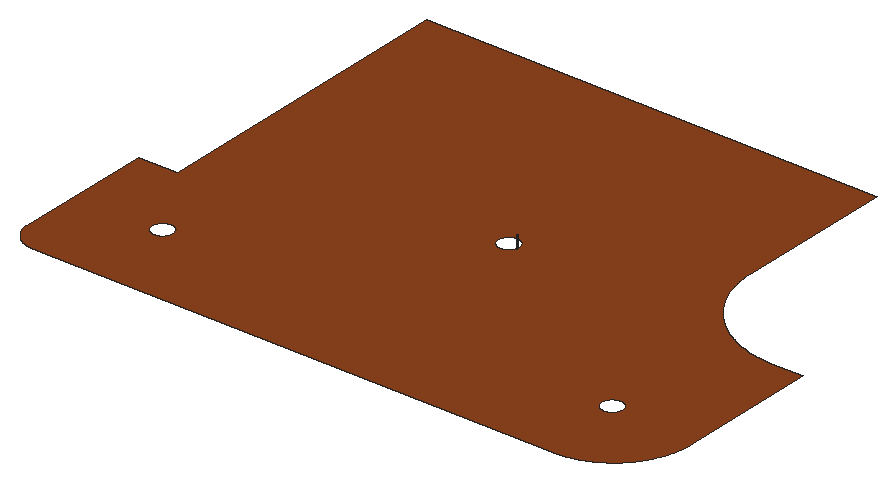
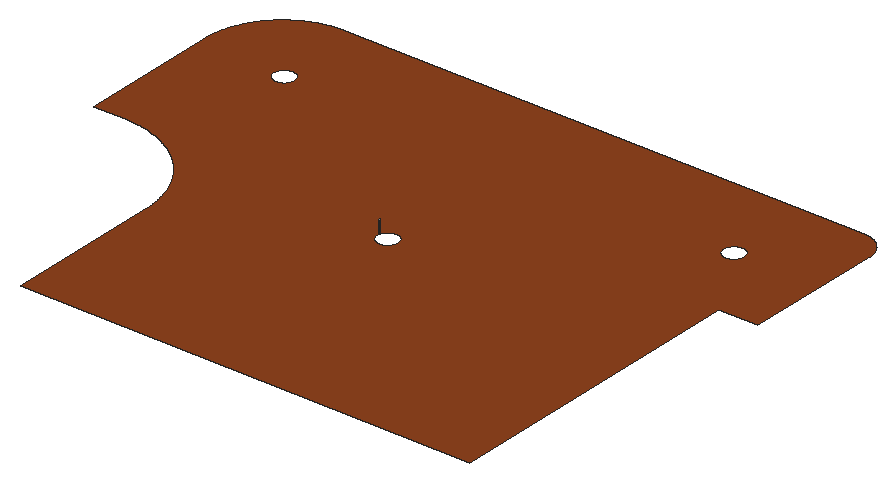
# SketchUp Ruby script. Lengths in inches.
U = 1.inch
M = Sketchup.active_model
def pt(a) = Geom::Point3d.new(a.map { |v| v * U })
def face(e, loops, mat)
  f = e.add_face(loops[0].map { |a| pt(a) })
  loops[1..].each { |l| e.add_face(l.map { |a| pt(a) }).erase! }
  f.material = f.back_material = mat if mat
  f
end
# faces: each face lists its corners as indices into pts; further lists are holes
def faces(e, pts, list, mat = nil) = list.each { |f| face(e, (f[0].is_a?(Array) ? f : [f]).map { |l| l.map { |i| pts[i] } }, mat) }
# xy, xz, yz: faces in a plane at the given z, y or x. An outline is a flat list of corners, or four numbers for a rectangle; further outlines are holes
def ring(l) = l.size == 4 ? [[l[0], l[1]], [l[2], l[1]], [l[2], l[3]], [l[0], l[3]]] : l.each_slice(2).to_a
def flat(e, list, mat, &to3) = list.each { |f| face(e, (f[0].is_a?(Array) ? f : [f]).map { |l| ring(l).map { |u, v| to3.(u, v) } }, mat) }
def xy(e, z, list, mat = nil) = flat(e, list, mat) { |x, y| [x, y, z] }
def xz(e, y, list, mat = nil) = flat(e, list, mat) { |x, z| [x, y, z] }
def yz(e, x, list, mat = nil) = flat(e, list, mat) { |y, z| [x, y, z] }
def lines(e, pts, list) = list.each { |a, b| e.add_line(pt(pts[a]), pt(pts[b])) }
# prism: a flat outline (further loops are holes) pulled along v
def prism(e, loops, v, mat = nil)
  f = face(e, loops, mat); d = Geom::Vector3d.new(v.map { |x| x * U })
  f.pushpull(f.normal.samedirection?(d) ? d.length : -d.length)
end
def box(e, o, s, mat = nil) = prism(e, [[o, [o[0] + s[0], o[1], o[2]], [o[0] + s[0], o[1] + s[1], o[2]], [o[0], o[1] + s[1], o[2]]]], [0, 0, s[2]], mat)
def at(x, y, z, deg = 0) = Geom::Transformation.translation(pt([x, y, z])) * Geom::Transformation.rotation(ORIGIN, Z_AXIS, deg.degrees)
def axes(o, x, y, z) = Geom::Transformation.new([*x, 0, *y, 0, *z, 0, *pt(o).to_a, 1])
def part(name) = M.definitions.add(name)
# library, detail: a bought-in or finely detailed component or shape, given as its bounding box
def library(name, o, s) = part(name).tap { |d| box(d.entities, o, s) }
def detail(e, o, s) = box(e.add_group.entities, o, s)
def put(e, d, t, mat = nil) = e.add_instance(d, t).tap { |i| i.material = mat if mat }
def group(e, t, mat = nil) = e.add_group.tap { |g| g.transformation = t; g.material = mat if mat }.entities
root = M.entities
M.materials.add("[Wood Fence]").color = [142, 67, 30]
xy(root,242,[[[21.02,135.92,20.92,135.93,20.6875,135.93,20.61,135.9375,20.53,135.94,20.29,135.97,20.22,135.98,20.14,135.99,20.0625,136,19.98,136.01,19.91,136.02,19.75,136.06,19.68,136.07,19.52,136.11,19.45,136.13,19.37,136.15,19.3,136.17,19.22,136.19,19.15,136.22,19.07,136.24,19,136.27,18.92,136.3,18.85,136.32,18.78,136.35,18.7,136.38,18.56,136.44,18.49,136.48,18.35,136.54,18.28,136.58,18.21,136.61,17.93,136.77,17.87,136.81,17.73,136.89,17.67,136.9375,17.6,136.98,17.54,137.02,17.47,137.07,17.41,137.12,17.35,137.16,17.29,137.21,17.22,137.26,17.16,137.3125,17.1,137.36,17.04,137.41,16.99,137.47,16.87,137.57,16.8125,137.625,16.76,137.68,16.59,137.85,16.49,137.97,16.4375,138.03,16.39,138.09,16.19,138.33,16.15,138.4,16.1,138.46,16.06,138.53,16.01,138.59,15.97,138.66,15.93,138.72,15.88,138.79,15.84,138.86,15.8,138.92,15.77,138.99,15.73,139.0625,15.69,139.13,15.65,139.2,15.62,139.27,15.58,139.34,15.52,139.48,15.49,139.56,15.4,139.77,15.37,139.85,15.34,139.92,15.32,140,15.29,140.07,15.27,140.15,15.25,140.22,15.23,140.3,15.2,140.37,15.18,140.45,15.17,140.52,15.13,140.68,15.12,140.75,15.1,140.83,15.09,140.91,15.07,140.99,15.0625,141.0625,15.05,141.14,15.03,141.3,15.03,141.375,15.02,141.45,15.01,141.53,15.01,141.61,15,141.6875,15,174,24,174,24,246,128,246,128,209.71,128.04,208.55,128.0625,208.26,128.09,207.97,128.11,207.68,128.14,207.4,128.17,207.11,128.25,206.53,128.3,206.25,128.34,205.96,128.39,205.67,128.45,205.39,128.5,205.1,128.57,204.82,128.63,204.54,128.77,203.98,128.84,203.69,128.92,203.42,129,203.14,129.09,202.86,129.17,202.58,129.27,202.31,129.36,202.03,129.66,201.22,129.88,200.68,130,200.42,130.11,200.15,130.23,199.89,130.49,199.36,130.62,199.1,130.75,198.85,130.89,198.59,131.02,198.34,131.17,198.08,131.3125,197.83,131.46,197.58,131.61,197.34,131.77,197.09,131.92,196.85,132.08,196.61,132.25,196.37,132.41,196.13,132.58,195.89,132.76,195.66,132.93,195.43,133.29,194.97,133.47,194.75,133.66,194.52,133.84,194.3,134.04,194.08,134.23,193.87,134.43,193.66,134.625,193.44,134.83,193.24,135.03,193.03,135.24,192.83,135.44,192.625,135.66,192.43,135.87,192.23,136.08,192.04,136.3,191.84,136.52,191.66,136.75,191.47,136.97,191.29,137.43,190.93,137.66,190.76,137.89,190.58,138.13,190.41,138.37,190.25,138.61,190.08,138.85,189.92,139.09,189.77,139.34,189.61,139.58,189.46,139.83,189.3125,140.08,189.17,140.34,189.02,140.59,188.89,140.85,188.75,141.1,188.62,141.36,188.49,141.89,188.23,142.15,188.11,142.42,188,142.68,187.88,143.22,187.66,144.03,187.36,144.31,187.27,144.58,187.17,144.86,187.09,145.14,187,145.42,186.92,145.69,186.84,145.98,186.77,146.54,186.63,146.82,186.57,147.1,186.5,147.39,186.45,147.67,186.39,147.96,186.34,148.25,186.3,148.53,186.25,149.11,186.17,149.4,186.14,149.68,186.11,149.97,186.09,150.26,186.0625,150.55,186.04,151.71,186,159,186,159,153.71,158.99,153.49,158.99,153.27,158.98,153.06,158.97,152.84,158.95,152.62,158.94,152.4,158.92,152.1875,158.89,151.97,158.87,151.76,158.84,151.54,158.8125,151.32,158.78,151.11,158.74,150.89,158.66,150.47,158.62,150.25,158.58,150.04,158.48,149.62,158.42,149.41,158.37,149.2,158.25,148.78,158.18,148.57,158.12,148.36,158.05,148.16,157.98,147.95,157.91,147.75,157.83,147.54,157.67,147.14,157.59,146.9375,157.5,146.74,157.23,146.14,157.14,145.95,157.04,145.75,156.9375,145.56,156.84,145.37,156.73,145.18,156.625,144.99,156.51,144.8,156.4,144.61,156.29,144.43,156.17,144.24,156.06,144.06,155.94,143.88,155.8125,143.7,155.5625,143.34,155.43,143.17,155.3,143,155.17,142.82,155.03,142.65,154.9,142.48,154.76,142.32,154.62,142.15,154.47,141.99,154.33,141.83,153.88,141.35,153.42,140.89,153.26,140.74,153.1,140.6,152.94,140.45,152.77,140.31,152.61,140.17,152.4375,140.03,152.27,139.89,152.1,139.76,151.93,139.62,151.75,139.49,151.58,139.36,151.4,139.24,151.22,139.11,150.5,138.63,149.75,138.19,149.56,138.09,149.36,137.99,148.98,137.79,148.78,137.69,148.58,137.6,148.39,137.51,148.1875,137.42,147.99,137.34,147.79,137.25,147.58,137.17,147.38,137.09,147.18,137.02,146.97,136.94,146.77,136.875,146.5625,136.81,146.35,136.74,146.15,136.68,145.9375,136.62,145.73,136.56,145.52,136.5,145.31,136.45,145.09,136.4,144.67,136.3,144.46,136.26,144.24,136.22,144.03,136.18,143.8125,136.15,143.6,136.11,143.38,136.08,143.17,136.06,142.95,136.03,142.74,136.01,142.3,135.97,142.09,135.96,141.87,135.95,141.65,135.9375,141.43,135.93,141.22,135.93,140.98,135.92],[86.84,188.5,87.16,188.5,87.24,188.51,87.3125,188.52,87.39,188.53,87.47,188.54,87.55,188.56,87.62,188.58,87.7,188.6,87.77,188.62,87.85,188.65,87.99,188.71,88.0625,188.74,88.13,188.77,88.41,188.93,88.47,188.98,88.53,189.02,88.59,189.07,88.71,189.18,88.77,189.23,88.82,189.29,88.93,189.41,88.98,189.47,89.02,189.53,89.07,189.59,89.23,189.87,89.26,189.9375,89.29,190.01,89.35,190.15,89.38,190.23,89.4,190.3,89.42,190.38,89.44,190.45,89.46,190.53,89.47,190.61,89.48,190.6875,89.49,190.76,89.5,190.84,89.5,191.16,89.49,191.24,89.48,191.3125,89.47,191.39,89.46,191.47,89.44,191.55,89.42,191.62,89.4,191.7,89.38,191.77,89.35,191.85,89.29,191.99,89.26,192.0625,89.23,192.13,89.07,192.41,89.02,192.47,88.98,192.53,88.93,192.59,88.82,192.71,88.77,192.77,88.71,192.82,88.59,192.93,88.53,192.98,88.47,193.02,88.41,193.07,88.13,193.23,88.0625,193.26,87.99,193.29,87.85,193.35,87.77,193.38,87.7,193.4,87.62,193.42,87.55,193.44,87.47,193.46,87.39,193.47,87.3125,193.48,87.24,193.49,87.16,193.5,86.84,193.5,86.76,193.49,86.6875,193.48,86.61,193.47,86.53,193.46,86.45,193.44,86.38,193.42,86.3,193.4,86.23,193.38,86.15,193.35,86.01,193.29,85.9375,193.26,85.87,193.23,85.59,193.07,85.53,193.02,85.47,192.98,85.41,192.93,85.29,192.82,85.23,192.77,85.18,192.71,85.07,192.59,85.02,192.53,84.98,192.47,84.93,192.41,84.77,192.13,84.74,192.0625,84.71,191.99,84.65,191.85,84.62,191.77,84.6,191.7,84.58,191.62,84.56,191.55,84.54,191.47,84.53,191.39,84.52,191.3125,84.51,191.24,84.5,191.16,84.5,190.84,84.51,190.76,84.52,190.6875,84.53,190.61,84.54,190.53,84.56,190.45,84.58,190.38,84.6,190.3,84.62,190.23,84.65,190.15,84.71,190.01,84.74,189.9375,84.77,189.87,84.93,189.59,84.98,189.53,85.02,189.47,85.07,189.41,85.18,189.29,85.23,189.23,85.29,189.18,85.41,189.07,85.47,189.02,85.53,188.98,85.59,188.93,85.87,188.77,85.9375,188.74,86.01,188.71,86.15,188.65,86.23,188.62,86.3,188.6,86.38,188.58,86.45,188.56,86.53,188.54,86.61,188.53,86.6875,188.52,86.76,188.51],[139,153.42,139.08,153.43,139.16,153.43,139.24,153.44,139.3125,153.44,139.39,153.46,139.55,153.48,139.62,153.5,139.7,153.52,139.77,153.55,139.85,153.57,139.99,153.63,140.0625,153.66,140.13,153.7,140.2,153.73,140.27,153.77,140.34,153.8125,140.41,153.86,140.47,153.9,140.71,154.1,140.82,154.21,140.93,154.33,140.98,154.39,141.02,154.45,141.07,154.52,141.11,154.58,141.23,154.79,141.32,155,141.35,155.08,141.38,155.15,141.4,155.23,141.42,155.3,141.46,155.46,141.47,155.53,141.48,155.61,141.49,155.6875,141.5,155.77,141.5,156.08,141.47,156.32,141.46,156.39,141.42,156.55,141.4,156.62,141.38,156.7,141.32,156.84,141.29,156.92,141.23,157.06,141.15,157.2,141.11,157.26,141.07,157.33,141.02,157.39,140.98,157.46,140.93,157.52,140.82,157.64,140.71,157.75,140.47,157.95,140.41,157.99,140.34,158.04,140.2,158.12,140.13,158.15,140.0625,158.1875,139.99,158.22,139.85,158.28,139.77,158.3,139.7,158.33,139.62,158.35,139.55,158.36,139.47,158.38,139.39,158.39,139.3125,158.4,139.24,158.41,139.16,158.42,138.84,158.42,138.76,158.41,138.6875,158.4,138.61,158.39,138.53,158.38,138.45,158.36,138.38,158.35,138.3,158.33,138.23,158.3,138.15,158.28,138.01,158.22,137.9375,158.1875,137.87,158.15,137.8,158.12,137.66,158.04,137.59,157.99,137.53,157.95,137.29,157.75,137.18,157.64,137.07,157.52,137.02,157.46,136.98,157.39,136.93,157.33,136.89,157.26,136.85,157.2,136.77,157.06,136.71,156.92,136.68,156.84,136.62,156.7,136.6,156.62,136.58,156.55,136.54,156.39,136.53,156.32,136.5,156.08,136.5,155.77,136.51,155.6875,136.52,155.61,136.53,155.53,136.54,155.46,136.58,155.3,136.6,155.23,136.62,155.15,136.65,155.08,136.68,155,136.77,154.79,136.89,154.58,136.93,154.52,136.98,154.45,137.02,154.39,137.07,154.33,137.18,154.21,137.29,154.1,137.53,153.9,137.59,153.86,137.66,153.8125,137.73,153.77,137.8,153.73,137.87,153.7,137.9375,153.66,138.01,153.63,138.15,153.57,138.23,153.55,138.3,153.52,138.38,153.5,138.45,153.48,138.61,153.46,138.6875,153.44,138.76,153.44,138.84,153.43,138.92,153.43],[35,153.42,35.08,153.43,35.16,153.43,35.24,153.44,35.3125,153.44,35.39,153.46,35.55,153.48,35.62,153.5,35.7,153.52,35.77,153.55,35.85,153.57,36.06,153.66,36.2,153.73,36.27,153.77,36.34,153.8125,36.41,153.86,36.47,153.9,36.71,154.1,36.82,154.21,36.93,154.33,36.98,154.39,37.02,154.45,37.07,154.52,37.11,154.58,37.23,154.79,37.32,155,37.35,155.08,37.38,155.15,37.4,155.23,37.42,155.3,37.46,155.46,37.47,155.53,37.48,155.61,37.49,155.6875,37.5,155.77,37.5,156.08,37.47,156.32,37.46,156.39,37.42,156.55,37.4,156.62,37.38,156.7,37.32,156.84,37.29,156.92,37.23,157.06,37.15,157.2,37.11,157.26,37.07,157.33,37.02,157.39,36.98,157.46,36.93,157.52,36.82,157.64,36.71,157.75,36.47,157.95,36.41,157.99,36.34,158.04,36.2,158.12,36.14,158.15,36.06,158.1875,35.99,158.22,35.85,158.28,35.77,158.3,35.7,158.33,35.62,158.35,35.55,158.36,35.47,158.38,35.39,158.39,35.3125,158.4,35.24,158.41,35.16,158.42,34.84,158.42,34.76,158.41,34.6875,158.4,34.61,158.39,34.53,158.38,34.45,158.36,34.38,158.35,34.3,158.33,34.23,158.3,34.15,158.28,34.01,158.22,33.9375,158.1875,33.87,158.15,33.8,158.12,33.66,158.04,33.59,157.99,33.53,157.95,33.29,157.75,33.18,157.64,33.07,157.52,33.02,157.46,32.98,157.39,32.93,157.33,32.89,157.26,32.85,157.2,32.77,157.06,32.71,156.92,32.68,156.84,32.62,156.7,32.6,156.62,32.58,156.55,32.54,156.39,32.53,156.32,32.51,156.16,32.51,156.08,32.5,156,32.5,155.85,32.51,155.77,32.51,155.6875,32.52,155.61,32.53,155.53,32.54,155.46,32.58,155.3,32.6,155.23,32.62,155.15,32.65,155.08,32.68,155,32.77,154.79,32.89,154.58,32.93,154.52,32.98,154.45,33.02,154.39,33.07,154.33,33.18,154.21,33.29,154.1,33.53,153.9,33.59,153.86,33.66,153.8125,33.73,153.77,33.8,153.73,33.87,153.7,33.9375,153.66,34.01,153.63,34.15,153.57,34.23,153.55,34.3,153.52,34.38,153.5,34.45,153.48,34.61,153.46,34.6875,153.44,34.76,153.44,34.84,153.43,34.92,153.43]]],"[Wood Fence]")
p = [[89.4,190.3,242],[89.38,190.23,242],[89.38,190.23,245],[89.4,190.3,245],[89.42,190.38,242],[89.42,190.38,245],
  [89.44,190.45,242],[89.44,190.45,245]]
faces(root,p,[[0,1,2,3],[4,0,3,5],[6,4,5,7]])
